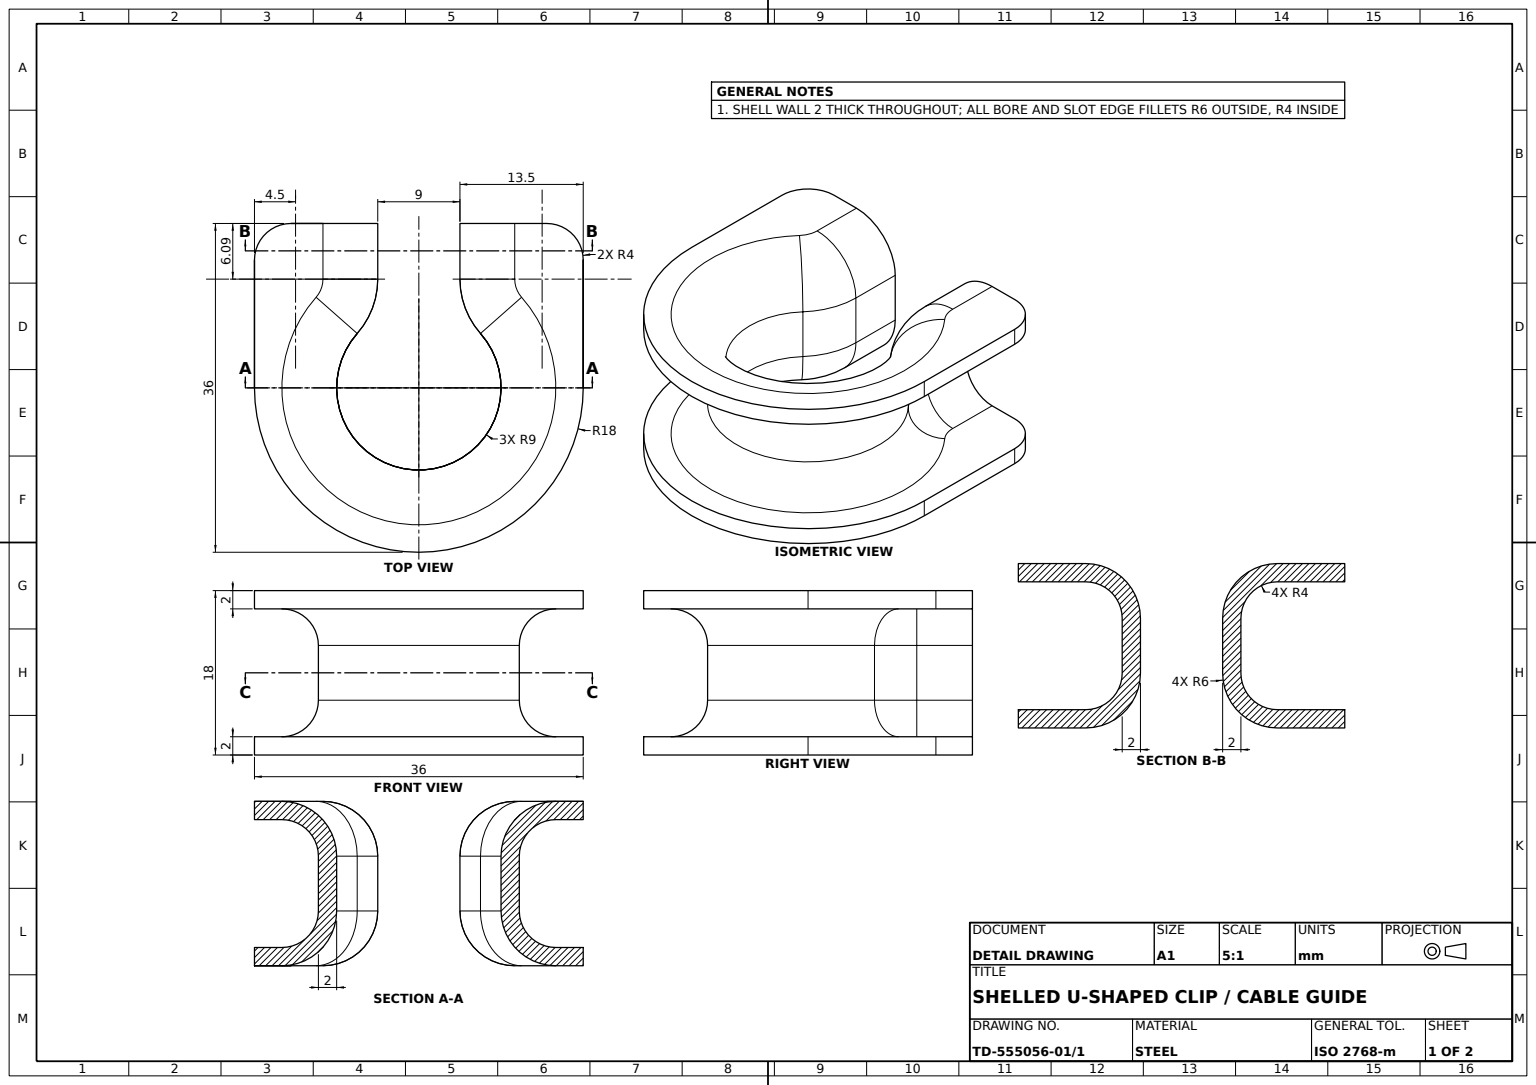
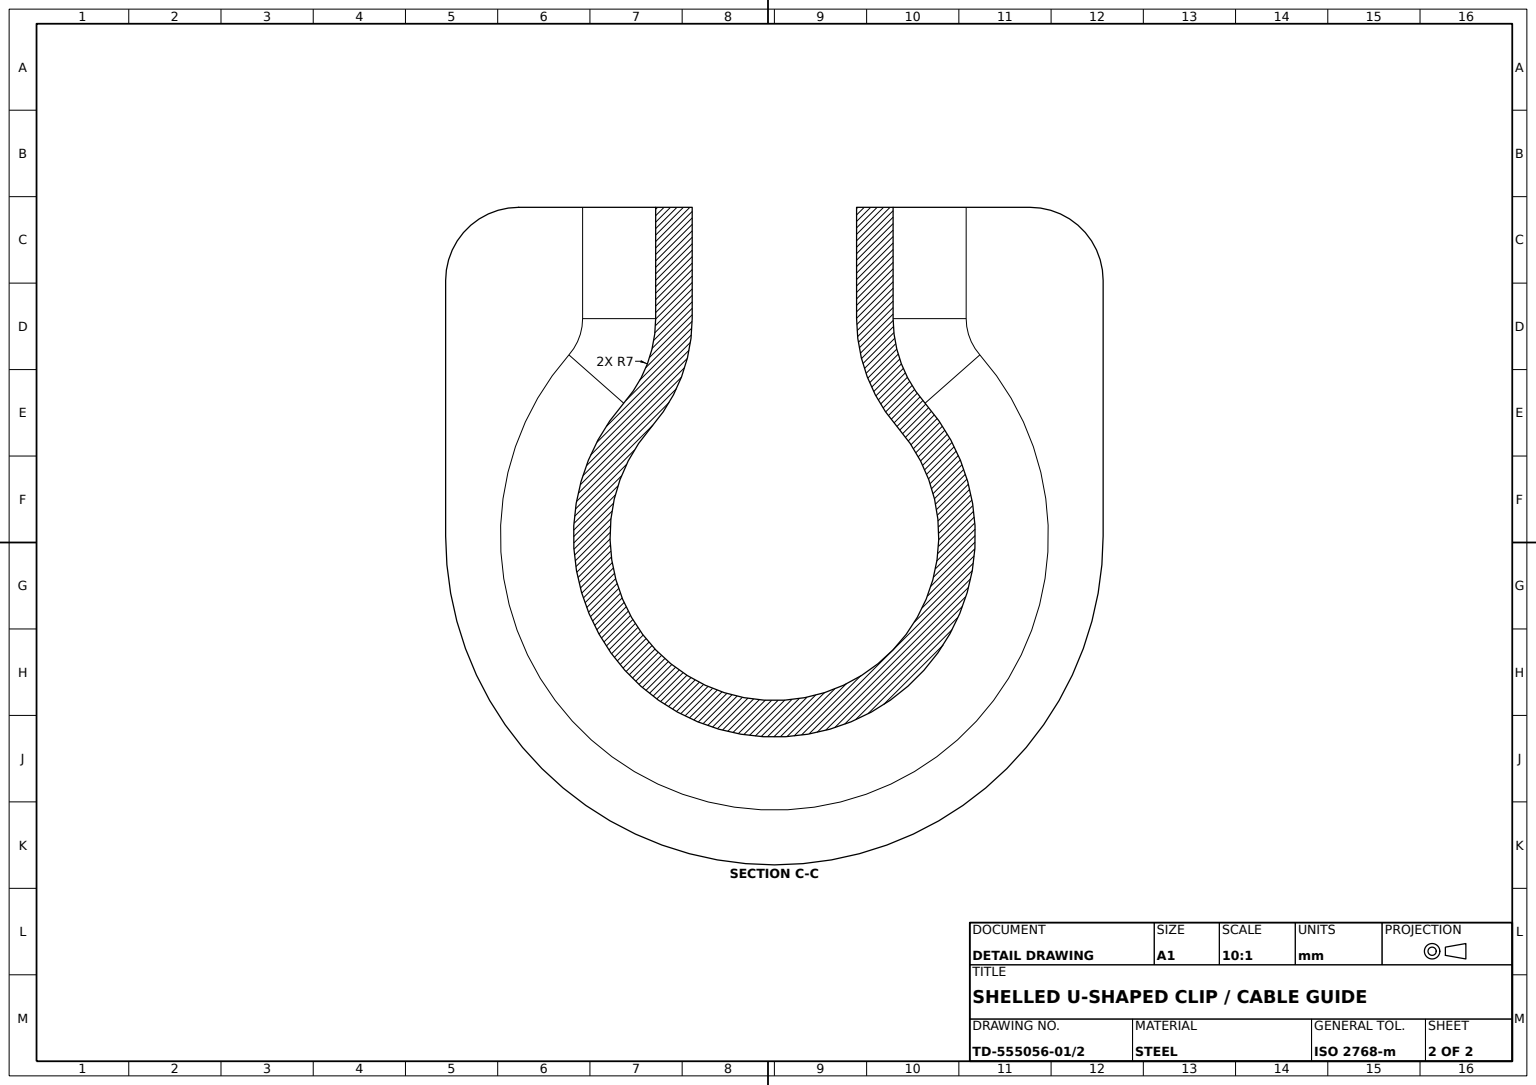
ISO-10303-21;
HEADER;
FILE_DESCRIPTION((''),'2;1');
FILE_NAME('','',(''),(''),'','','');
FILE_SCHEMA(('AUTOMOTIVE_DESIGN'));
ENDSEC;
DATA;
#1=APPLICATION_CONTEXT('');
#2=PRODUCT_CONTEXT('',#1,'mechanical');
#3=PRODUCT('','','',(#2));
#4=PRODUCT_DEFINITION_FORMATION('','',#3);
#5=PRODUCT_DEFINITION_CONTEXT('',#1,'design');
#6=PRODUCT_DEFINITION('','',#4,#5);
#7=PRODUCT_DEFINITION_SHAPE('','',#6);
#8=(LENGTH_UNIT()NAMED_UNIT(*)SI_UNIT(.MILLI.,.METRE.));
#9=(NAMED_UNIT(*)PLANE_ANGLE_UNIT()SI_UNIT($,.RADIAN.));
#10=(NAMED_UNIT(*)SI_UNIT($,.STERADIAN.)SOLID_ANGLE_UNIT());
#11=UNCERTAINTY_MEASURE_WITH_UNIT(LENGTH_MEASURE(1.E-05),#8,'distance_accuracy_value','');
#12=(GEOMETRIC_REPRESENTATION_CONTEXT(3)GLOBAL_UNCERTAINTY_ASSIGNED_CONTEXT((#11))GLOBAL_UNIT_ASSIGNED_CONTEXT((#8,#9,#10))REPRESENTATION_CONTEXT('',''));
#13=CARTESIAN_POINT('',(8.25,-3.,-7.275816));
#14=VERTEX_POINT('',#13);
#15=CARTESIAN_POINT('',(-8.25,-3.,-7.275816));
#16=VERTEX_POINT('',#15);
#17=CARTESIAN_POINT('',(0.,-3.,0.));
#18=DIRECTION('',(0.,-1.,0.));
#19=DIRECTION('',(0.,0.,-1.));
#20=AXIS2_PLACEMENT_3D('',#17,#18,#19);
#21=CIRCLE('',#20,11.);
#22=EDGE_CURVE('',#14,#16,#21,.T.);
#23=ORIENTED_EDGE('',*,*,#22,.F.);
#24=CARTESIAN_POINT('',(8.25,3.,-7.275816));
#25=VERTEX_POINT('',#24);
#26=CARTESIAN_POINT('',(8.25,9.,-7.275816));
#27=VECTOR('',#18,1000.);
#28=LINE('',#26,#27);
#29=EDGE_CURVE('',#25,#14,#28,.T.);
#30=ORIENTED_EDGE('',*,*,#29,.F.);
#31=CARTESIAN_POINT('',(-8.25,3.,-7.275816));
#32=VERTEX_POINT('',#31);
#33=CARTESIAN_POINT('',(0.,3.,0.));
#34=DIRECTION('',(0.,1.,0.));
#35=AXIS2_PLACEMENT_3D('',#33,#34,#19);
#36=CIRCLE('',#35,11.);
#37=EDGE_CURVE('',#32,#25,#36,.T.);
#38=ORIENTED_EDGE('',*,*,#37,.F.);
#39=CARTESIAN_POINT('',(-8.25,9.,-7.275816));
#40=LINE('',#39,#27);
#41=EDGE_CURVE('',#32,#16,#40,.T.);
#42=ORIENTED_EDGE('',*,*,#41,.T.);
#43=EDGE_LOOP('',(#23,#30,#38,#42));
#44=FACE_OUTER_BOUND('',#43,.T.);
#45=CARTESIAN_POINT('',(0.,9.,0.));
#46=AXIS2_PLACEMENT_3D('',#45,#18,#19);
#47=CYLINDRICAL_SURFACE('',#46,11.);
#48=ADVANCED_FACE('',(#44),#47,.T.);
#49=CARTESIAN_POINT('',(4.5,-3.,-11.905881));
#50=VERTEX_POINT('',#49);
#51=CARTESIAN_POINT('',(6.75,-3.,-5.95294));
#52=VERTEX_POINT('',#51);
#53=CARTESIAN_POINT('',(13.5,-3.,-11.905881));
#54=AXIS2_PLACEMENT_3D('',#53,#34,#19);
#55=CIRCLE('',#54,9.);
#56=EDGE_CURVE('',#50,#52,#55,.T.);
#57=ORIENTED_EDGE('',*,*,#56,.T.);
#58=CARTESIAN_POINT('',(6.75,3.,-5.95294));
#59=VERTEX_POINT('',#58);
#60=CARTESIAN_POINT('',(6.75,9.,-5.95294));
#61=LINE('',#60,#27);
#62=EDGE_CURVE('',#59,#52,#61,.T.);
#63=ORIENTED_EDGE('',*,*,#62,.F.);
#64=CARTESIAN_POINT('',(4.5,3.,-11.905881));
#65=VERTEX_POINT('',#64);
#66=CARTESIAN_POINT('',(13.5,3.,-11.905881));
#67=AXIS2_PLACEMENT_3D('',#66,#18,#19);
#68=CIRCLE('',#67,9.);
#69=EDGE_CURVE('',#59,#65,#68,.T.);
#70=ORIENTED_EDGE('',*,*,#69,.T.);
#71=CARTESIAN_POINT('',(4.5,9.,-11.905881));
#72=LINE('',#71,#27);
#73=EDGE_CURVE('',#65,#50,#72,.T.);
#74=ORIENTED_EDGE('',*,*,#73,.T.);
#75=EDGE_LOOP('',(#57,#63,#70,#74));
#76=FACE_OUTER_BOUND('',#75,.T.);
#77=CARTESIAN_POINT('',(13.5,9.,-11.905881));
#78=AXIS2_PLACEMENT_3D('',#77,#18,#19);
#79=CYLINDRICAL_SURFACE('',#78,9.);
#80=ADVANCED_FACE('',(#76),#79,.T.);
#81=CARTESIAN_POINT('',(4.5,-3.,-18.));
#82=VERTEX_POINT('',#81);
#83=DIRECTION('',(0.,0.,1.));
#84=VECTOR('',#83,1000.);
#85=LINE('',#49,#84);
#86=EDGE_CURVE('',#82,#50,#85,.T.);
#87=ORIENTED_EDGE('',*,*,#86,.T.);
#88=ORIENTED_EDGE('',*,*,#73,.F.);
#89=CARTESIAN_POINT('',(4.5,3.,-18.));
#90=VERTEX_POINT('',#89);
#91=VECTOR('',#19,1000.);
#92=LINE('',#89,#91);
#93=EDGE_CURVE('',#65,#90,#92,.T.);
#94=ORIENTED_EDGE('',*,*,#93,.T.);
#95=CARTESIAN_POINT('',(4.5,9.,-18.));
#96=LINE('',#95,#27);
#97=EDGE_CURVE('',#90,#82,#96,.T.);
#98=ORIENTED_EDGE('',*,*,#97,.T.);
#99=EDGE_LOOP('',(#87,#88,#94,#98));
#100=FACE_OUTER_BOUND('',#99,.T.);
#101=DIRECTION('',(1.,0.,0.));
#102=AXIS2_PLACEMENT_3D('',#95,#101,#19);
#103=PLANE('',#102);
#104=ADVANCED_FACE('',(#100),#103,.F.);
#105=CARTESIAN_POINT('',(-4.5,3.,-11.905881));
#106=VERTEX_POINT('',#105);
#107=CARTESIAN_POINT('',(-6.75,3.,-5.95294));
#108=VERTEX_POINT('',#107);
#109=CARTESIAN_POINT('',(-13.5,3.,-11.905881));
#110=AXIS2_PLACEMENT_3D('',#109,#18,#19);
#111=CIRCLE('',#110,9.);
#112=EDGE_CURVE('',#106,#108,#111,.T.);
#113=ORIENTED_EDGE('',*,*,#112,.F.);
#114=CARTESIAN_POINT('',(-10.5,9.,-11.905881));
#115=VERTEX_POINT('',#114);
#116=CARTESIAN_POINT('',(-10.5,3.,-11.905881));
#117=AXIS2_PLACEMENT_3D('',#116,#83,#101);
#118=CIRCLE('',#117,6.);
#119=EDGE_CURVE('',#106,#115,#118,.T.);
#120=ORIENTED_EDGE('',*,*,#119,.T.);
#121=CARTESIAN_POINT('',(-11.25,9.,-9.921567));
#122=VERTEX_POINT('',#121);
#123=CARTESIAN_POINT('',(-13.5,9.,-11.905881));
#124=AXIS2_PLACEMENT_3D('',#123,#34,#19);
#125=CIRCLE('',#124,3.);
#126=EDGE_CURVE('',#122,#115,#125,.T.);
#127=ORIENTED_EDGE('',*,*,#126,.F.);
#128=CARTESIAN_POINT('',(-11.25,3.,-9.921567));
#129=DIRECTION('',(-0.661437828,0.,0.75));
#130=DIRECTION('',(0.75,0.,0.661437828));
#131=AXIS2_PLACEMENT_3D('',#128,#129,#130);
#132=CIRCLE('',#131,6.);
#133=EDGE_CURVE('',#108,#122,#132,.T.);
#134=ORIENTED_EDGE('',*,*,#133,.F.);
#135=EDGE_LOOP('',(#113,#120,#127,#134));
#136=FACE_OUTER_BOUND('',#135,.T.);
#137=TOROIDAL_SURFACE('',#110,3.,6.);
#138=ADVANCED_FACE('',(#136),#137,.T.);
#139=CARTESIAN_POINT('',(10.5,-9.,-11.905881));
#140=VERTEX_POINT('',#139);
#141=CARTESIAN_POINT('',(10.5,-9.,-18.));
#142=VERTEX_POINT('',#141);
#143=LINE('',#141,#91);
#144=EDGE_CURVE('',#140,#142,#143,.T.);
#145=ORIENTED_EDGE('',*,*,#144,.F.);
#146=CARTESIAN_POINT('',(10.5,-3.,-11.905881));
#147=DIRECTION('',(-1.,0.,0.));
#148=AXIS2_PLACEMENT_3D('',#146,#19,#147);
#149=CIRCLE('',#148,6.);
#150=EDGE_CURVE('',#140,#50,#149,.T.);
#151=ORIENTED_EDGE('',*,*,#150,.T.);
#152=ORIENTED_EDGE('',*,*,#86,.F.);
#153=CARTESIAN_POINT('',(10.5,-3.,-18.));
#154=AXIS2_PLACEMENT_3D('',#153,#19,#101);
#155=CIRCLE('',#154,6.);
#156=EDGE_CURVE('',#142,#82,#155,.T.);
#157=ORIENTED_EDGE('',*,*,#156,.F.);
#158=EDGE_LOOP('',(#145,#151,#152,#157));
#159=FACE_OUTER_BOUND('',#158,.T.);
#160=AXIS2_PLACEMENT_3D('',#153,#19,#147);
#161=CYLINDRICAL_SURFACE('',#160,6.);
#162=ADVANCED_FACE('',(#159),#161,.T.);
#163=CARTESIAN_POINT('',(-18.,7.,0.));
#164=VERTEX_POINT('',#163);
#165=CARTESIAN_POINT('',(18.,7.,0.));
#166=VERTEX_POINT('',#165);
#167=CARTESIAN_POINT('',(0.,7.,0.));
#168=AXIS2_PLACEMENT_3D('',#167,#34,#19);
#169=CIRCLE('',#168,18.);
#170=EDGE_CURVE('',#164,#166,#169,.T.);
#171=ORIENTED_EDGE('',*,*,#170,.T.);
#172=CARTESIAN_POINT('',(18.,9.,0.));
#173=VERTEX_POINT('',#172);
#174=LINE('',#172,#27);
#175=EDGE_CURVE('',#173,#166,#174,.T.);
#176=ORIENTED_EDGE('',*,*,#175,.F.);
#177=CARTESIAN_POINT('',(-18.,9.,0.));
#178=VERTEX_POINT('',#177);
#179=AXIS2_PLACEMENT_3D('',#45,#34,#83);
#180=CIRCLE('',#179,18.);
#181=EDGE_CURVE('',#178,#173,#180,.T.);
#182=ORIENTED_EDGE('',*,*,#181,.F.);
#183=LINE('',#177,#27);
#184=EDGE_CURVE('',#178,#164,#183,.T.);
#185=ORIENTED_EDGE('',*,*,#184,.T.);
#186=EDGE_LOOP('',(#171,#176,#182,#185));
#187=FACE_OUTER_BOUND('',#186,.T.);
#188=CYLINDRICAL_SURFACE('',#46,18.);
#189=ADVANCED_FACE('',(#187),#188,.T.);
#190=CARTESIAN_POINT('',(11.25,7.,-9.921567));
#191=VERTEX_POINT('',#190);
#192=CARTESIAN_POINT('',(-11.25,7.,-9.921567));
#193=VERTEX_POINT('',#192);
#194=AXIS2_PLACEMENT_3D('',#167,#18,#19);
#195=CIRCLE('',#194,15.);
#196=EDGE_CURVE('',#191,#193,#195,.T.);
#197=ORIENTED_EDGE('',*,*,#196,.T.);
#198=CIRCLE('',#131,4.);
#199=EDGE_CURVE('',#32,#193,#198,.T.);
#200=ORIENTED_EDGE('',*,*,#199,.F.);
#201=ORIENTED_EDGE('',*,*,#37,.T.);
#202=CARTESIAN_POINT('',(11.25,3.,-9.921567));
#203=DIRECTION('',(-0.661437828,0.,-0.75));
#204=DIRECTION('',(0.75,0.,-0.661437828));
#205=AXIS2_PLACEMENT_3D('',#202,#203,#204);
#206=CIRCLE('',#205,4.);
#207=EDGE_CURVE('',#25,#191,#206,.T.);
#208=ORIENTED_EDGE('',*,*,#207,.T.);
#209=EDGE_LOOP('',(#197,#200,#201,#208));
#210=FACE_OUTER_BOUND('',#209,.T.);
#211=AXIS2_PLACEMENT_3D('',#33,#18,#19);
#212=TOROIDAL_SURFACE('',#211,15.,4.);
#213=ADVANCED_FACE('',(#210),#212,.F.);
#214=CARTESIAN_POINT('',(6.5,3.,-11.905881));
#215=VERTEX_POINT('',#214);
#216=CARTESIAN_POINT('',(10.5,7.,-11.905881));
#217=VERTEX_POINT('',#216);
#218=CARTESIAN_POINT('',(10.5,3.,-11.905881));
#219=AXIS2_PLACEMENT_3D('',#218,#19,#101);
#220=CIRCLE('',#219,4.);
#221=EDGE_CURVE('',#215,#217,#220,.T.);
#222=ORIENTED_EDGE('',*,*,#221,.T.);
#223=CARTESIAN_POINT('',(13.5,7.,-11.905881));
#224=AXIS2_PLACEMENT_3D('',#223,#34,#19);
#225=CIRCLE('',#224,3.);
#226=EDGE_CURVE('',#217,#191,#225,.T.);
#227=ORIENTED_EDGE('',*,*,#226,.T.);
#228=ORIENTED_EDGE('',*,*,#207,.F.);
#229=CIRCLE('',#67,7.);
#230=EDGE_CURVE('',#25,#215,#229,.T.);
#231=ORIENTED_EDGE('',*,*,#230,.T.);
#232=EDGE_LOOP('',(#222,#227,#228,#231));
#233=FACE_OUTER_BOUND('',#232,.T.);
#234=TOROIDAL_SURFACE('',#67,3.,4.);
#235=ADVANCED_FACE('',(#233),#234,.F.);
#236=CARTESIAN_POINT('',(-6.5,-3.,-18.));
#237=VERTEX_POINT('',#236);
#238=CARTESIAN_POINT('',(-10.5,-7.,-18.));
#239=VERTEX_POINT('',#238);
#240=CARTESIAN_POINT('',(-10.5,-3.,-18.));
#241=AXIS2_PLACEMENT_3D('',#240,#19,#101);
#242=CIRCLE('',#241,4.);
#243=EDGE_CURVE('',#237,#239,#242,.T.);
#244=ORIENTED_EDGE('',*,*,#243,.F.);
#245=CARTESIAN_POINT('',(-6.5,3.,-18.));
#246=VERTEX_POINT('',#245);
#247=CARTESIAN_POINT('',(-6.5,9.,-18.));
#248=LINE('',#247,#27);
#249=EDGE_CURVE('',#246,#237,#248,.T.);
#250=ORIENTED_EDGE('',*,*,#249,.F.);
#251=CARTESIAN_POINT('',(-10.5,7.,-18.));
#252=VERTEX_POINT('',#251);
#253=CARTESIAN_POINT('',(-10.5,3.,-18.));
#254=AXIS2_PLACEMENT_3D('',#253,#19,#101);
#255=CIRCLE('',#254,4.);
#256=EDGE_CURVE('',#252,#246,#255,.T.);
#257=ORIENTED_EDGE('',*,*,#256,.F.);
#258=CARTESIAN_POINT('',(-14.,7.,-18.));
#259=VERTEX_POINT('',#258);
#260=CARTESIAN_POINT('',(-13.5,7.,-18.));
#261=VECTOR('',#147,1000.);
#262=LINE('',#260,#261);
#263=EDGE_CURVE('',#252,#259,#262,.T.);
#264=ORIENTED_EDGE('',*,*,#263,.T.);
#265=CARTESIAN_POINT('',(-14.,9.,-18.));
#266=VERTEX_POINT('',#265);
#267=LINE('',#265,#27);
#268=EDGE_CURVE('',#266,#259,#267,.T.);
#269=ORIENTED_EDGE('',*,*,#268,.F.);
#270=CARTESIAN_POINT('',(-10.5,9.,-18.));
#271=VERTEX_POINT('',#270);
#272=LINE('',#265,#261);
#273=EDGE_CURVE('',#271,#266,#272,.T.);
#274=ORIENTED_EDGE('',*,*,#273,.F.);
#275=CARTESIAN_POINT('',(-4.5,3.,-18.));
#276=VERTEX_POINT('',#275);
#277=CIRCLE('',#254,6.);
#278=EDGE_CURVE('',#271,#276,#277,.T.);
#279=ORIENTED_EDGE('',*,*,#278,.T.);
#280=CARTESIAN_POINT('',(-4.5,-3.,-18.));
#281=VERTEX_POINT('',#280);
#282=CARTESIAN_POINT('',(-4.5,9.,-18.));
#283=LINE('',#282,#27);
#284=EDGE_CURVE('',#276,#281,#283,.T.);
#285=ORIENTED_EDGE('',*,*,#284,.T.);
#286=CARTESIAN_POINT('',(-10.5,-9.,-18.));
#287=VERTEX_POINT('',#286);
#288=CIRCLE('',#241,6.);
#289=EDGE_CURVE('',#281,#287,#288,.T.);
#290=ORIENTED_EDGE('',*,*,#289,.T.);
#291=CARTESIAN_POINT('',(-14.,-9.,-18.));
#292=VERTEX_POINT('',#291);
#293=LINE('',#291,#261);
#294=EDGE_CURVE('',#287,#292,#293,.T.);
#295=ORIENTED_EDGE('',*,*,#294,.T.);
#296=CARTESIAN_POINT('',(-14.,-7.,-18.));
#297=VERTEX_POINT('',#296);
#298=EDGE_CURVE('',#297,#292,#267,.T.);
#299=ORIENTED_EDGE('',*,*,#298,.F.);
#300=CARTESIAN_POINT('',(-13.5,-7.,-18.));
#301=LINE('',#300,#261);
#302=EDGE_CURVE('',#239,#297,#301,.T.);
#303=ORIENTED_EDGE('',*,*,#302,.F.);
#304=EDGE_LOOP('',(#244,#250,#257,#264,#269,#274,#279,#285,#290,#295,#299,#303));
#305=FACE_OUTER_BOUND('',#304,.T.);
#306=AXIS2_PLACEMENT_3D('',#265,#83,#101);
#307=PLANE('',#306);
#308=ADVANCED_FACE('',(#305),#307,.F.);
#309=CARTESIAN_POINT('',(-6.5,3.,-11.905881));
#310=VERTEX_POINT('',#309);
#311=CIRCLE('',#110,7.);
#312=EDGE_CURVE('',#310,#32,#311,.T.);
#313=ORIENTED_EDGE('',*,*,#312,.F.);
#314=CARTESIAN_POINT('',(-6.5,-3.,-11.905881));
#315=VERTEX_POINT('',#314);
#316=CARTESIAN_POINT('',(-6.5,9.,-11.905881));
#317=LINE('',#316,#27);
#318=EDGE_CURVE('',#310,#315,#317,.T.);
#319=ORIENTED_EDGE('',*,*,#318,.T.);
#320=CARTESIAN_POINT('',(-13.5,-3.,-11.905881));
#321=AXIS2_PLACEMENT_3D('',#320,#34,#19);
#322=CIRCLE('',#321,7.);
#323=EDGE_CURVE('',#16,#315,#322,.T.);
#324=ORIENTED_EDGE('',*,*,#323,.F.);
#325=ORIENTED_EDGE('',*,*,#41,.F.);
#326=EDGE_LOOP('',(#313,#319,#324,#325));
#327=FACE_OUTER_BOUND('',#326,.T.);
#328=AXIS2_PLACEMENT_3D('',#123,#18,#19);
#329=CYLINDRICAL_SURFACE('',#328,7.);
#330=ADVANCED_FACE('',(#327),#329,.F.);
#331=CARTESIAN_POINT('',(10.5,-7.,-11.905881));
#332=VERTEX_POINT('',#331);
#333=CARTESIAN_POINT('',(10.5,-7.,-18.));
#334=VERTEX_POINT('',#333);
#335=LINE('',#331,#91);
#336=EDGE_CURVE('',#332,#334,#335,.T.);
#337=ORIENTED_EDGE('',*,*,#336,.F.);
#338=CARTESIAN_POINT('',(11.25,-7.,-9.921567));
#339=VERTEX_POINT('',#338);
#340=CARTESIAN_POINT('',(13.5,-7.,-11.905881));
#341=AXIS2_PLACEMENT_3D('',#340,#18,#19);
#342=CIRCLE('',#341,3.);
#343=EDGE_CURVE('',#339,#332,#342,.T.);
#344=ORIENTED_EDGE('',*,*,#343,.F.);
#345=CARTESIAN_POINT('',(-11.25,-7.,-9.921567));
#346=VERTEX_POINT('',#345);
#347=CARTESIAN_POINT('',(0.,-7.,0.));
#348=AXIS2_PLACEMENT_3D('',#347,#34,#19);
#349=CIRCLE('',#348,15.);
#350=EDGE_CURVE('',#346,#339,#349,.T.);
#351=ORIENTED_EDGE('',*,*,#350,.F.);
#352=CARTESIAN_POINT('',(-10.5,-7.,-11.905881));
#353=VERTEX_POINT('',#352);
#354=CARTESIAN_POINT('',(-13.5,-7.,-11.905881));
#355=AXIS2_PLACEMENT_3D('',#354,#18,#19);
#356=CIRCLE('',#355,3.);
#357=EDGE_CURVE('',#353,#346,#356,.T.);
#358=ORIENTED_EDGE('',*,*,#357,.F.);
#359=LINE('',#352,#84);
#360=EDGE_CURVE('',#239,#353,#359,.T.);
#361=ORIENTED_EDGE('',*,*,#360,.F.);
#362=ORIENTED_EDGE('',*,*,#302,.T.);
#363=CARTESIAN_POINT('',(-18.,-7.,-14.));
#364=VERTEX_POINT('',#363);
#365=CARTESIAN_POINT('',(-14.,-7.,-14.));
#366=AXIS2_PLACEMENT_3D('',#365,#34,#19);
#367=CIRCLE('',#366,4.);
#368=EDGE_CURVE('',#297,#364,#367,.T.);
#369=ORIENTED_EDGE('',*,*,#368,.T.);
#370=CARTESIAN_POINT('',(-18.,-7.,0.));
#371=VERTEX_POINT('',#370);
#372=CARTESIAN_POINT('',(-18.,-7.,-11.905881));
#373=LINE('',#372,#84);
#374=EDGE_CURVE('',#364,#371,#373,.T.);
#375=ORIENTED_EDGE('',*,*,#374,.T.);
#376=CARTESIAN_POINT('',(18.,-7.,0.));
#377=VERTEX_POINT('',#376);
#378=CIRCLE('',#348,18.);
#379=EDGE_CURVE('',#371,#377,#378,.T.);
#380=ORIENTED_EDGE('',*,*,#379,.T.);
#381=CARTESIAN_POINT('',(18.,-7.,-14.));
#382=VERTEX_POINT('',#381);
#383=CARTESIAN_POINT('',(18.,-7.,-11.905881));
#384=LINE('',#383,#91);
#385=EDGE_CURVE('',#377,#382,#384,.T.);
#386=ORIENTED_EDGE('',*,*,#385,.T.);
#387=CARTESIAN_POINT('',(14.,-7.,-18.));
#388=VERTEX_POINT('',#387);
#389=CARTESIAN_POINT('',(14.,-7.,-14.));
#390=AXIS2_PLACEMENT_3D('',#389,#34,#19);
#391=CIRCLE('',#390,4.);
#392=EDGE_CURVE('',#382,#388,#391,.T.);
#393=ORIENTED_EDGE('',*,*,#392,.T.);
#394=EDGE_CURVE('',#388,#334,#301,.T.);
#395=ORIENTED_EDGE('',*,*,#394,.T.);
#396=EDGE_LOOP('',(#337,#344,#351,#358,#361,#362,#369,#375,#380,#386,#393,#395));
#397=FACE_OUTER_BOUND('',#396,.T.);
#398=PLANE('',#355);
#399=ADVANCED_FACE('',(#397),#398,.F.);
#400=CARTESIAN_POINT('',(-10.5,-9.,-11.905881));
#401=VERTEX_POINT('',#400);
#402=LINE('',#400,#84);
#403=EDGE_CURVE('',#287,#401,#402,.T.);
#404=ORIENTED_EDGE('',*,*,#403,.F.);
#405=ORIENTED_EDGE('',*,*,#289,.F.);
#406=CARTESIAN_POINT('',(-4.5,-3.,-11.905881));
#407=VERTEX_POINT('',#406);
#408=LINE('',#280,#91);
#409=EDGE_CURVE('',#407,#281,#408,.T.);
#410=ORIENTED_EDGE('',*,*,#409,.F.);
#411=CARTESIAN_POINT('',(-10.5,-3.,-11.905881));
#412=AXIS2_PLACEMENT_3D('',#411,#83,#101);
#413=CIRCLE('',#412,6.);
#414=EDGE_CURVE('',#401,#407,#413,.T.);
#415=ORIENTED_EDGE('',*,*,#414,.F.);
#416=EDGE_LOOP('',(#404,#405,#410,#415));
#417=FACE_OUTER_BOUND('',#416,.T.);
#418=AXIS2_PLACEMENT_3D('',#240,#83,#101);
#419=CYLINDRICAL_SURFACE('',#418,6.);
#420=ADVANCED_FACE('',(#417),#419,.T.);
#421=ORIENTED_EDGE('',*,*,#69,.F.);
#422=CARTESIAN_POINT('',(11.25,9.,-9.921567));
#423=VERTEX_POINT('',#422);
#424=DIRECTION('',(-0.75,0.,0.661437828));
#425=AXIS2_PLACEMENT_3D('',#202,#203,#424);
#426=CIRCLE('',#425,6.);
#427=EDGE_CURVE('',#59,#423,#426,.T.);
#428=ORIENTED_EDGE('',*,*,#427,.T.);
#429=CARTESIAN_POINT('',(10.5,9.,-11.905881));
#430=VERTEX_POINT('',#429);
#431=AXIS2_PLACEMENT_3D('',#77,#34,#19);
#432=CIRCLE('',#431,3.);
#433=EDGE_CURVE('',#430,#423,#432,.T.);
#434=ORIENTED_EDGE('',*,*,#433,.F.);
#435=AXIS2_PLACEMENT_3D('',#218,#19,#147);
#436=CIRCLE('',#435,6.);
#437=EDGE_CURVE('',#65,#430,#436,.T.);
#438=ORIENTED_EDGE('',*,*,#437,.F.);
#439=EDGE_LOOP('',(#421,#428,#434,#438));
#440=FACE_OUTER_BOUND('',#439,.T.);
#441=TOROIDAL_SURFACE('',#67,3.,6.);
#442=ADVANCED_FACE('',(#440),#441,.T.);
#443=CARTESIAN_POINT('',(10.5,9.,-18.));
#444=VERTEX_POINT('',#443);
#445=LINE('',#429,#84);
#446=EDGE_CURVE('',#444,#430,#445,.T.);
#447=ORIENTED_EDGE('',*,*,#446,.F.);
#448=CARTESIAN_POINT('',(10.5,3.,-18.));
#449=AXIS2_PLACEMENT_3D('',#448,#19,#101);
#450=CIRCLE('',#449,6.);
#451=EDGE_CURVE('',#90,#444,#450,.T.);
#452=ORIENTED_EDGE('',*,*,#451,.F.);
#453=ORIENTED_EDGE('',*,*,#93,.F.);
#454=ORIENTED_EDGE('',*,*,#437,.T.);
#455=EDGE_LOOP('',(#447,#452,#453,#454));
#456=FACE_OUTER_BOUND('',#455,.T.);
#457=AXIS2_PLACEMENT_3D('',#218,#83,#101);
#458=CYLINDRICAL_SURFACE('',#457,6.);
#459=ADVANCED_FACE('',(#456),#458,.T.);
#460=ORIENTED_EDGE('',*,*,#385,.F.);
#461=CARTESIAN_POINT('',(18.,-9.,0.));
#462=VERTEX_POINT('',#461);
#463=EDGE_CURVE('',#377,#462,#174,.T.);
#464=ORIENTED_EDGE('',*,*,#463,.T.);
#465=CARTESIAN_POINT('',(18.,-9.,-14.));
#466=VERTEX_POINT('',#465);
#467=LINE('',#465,#91);
#468=EDGE_CURVE('',#462,#466,#467,.T.);
#469=ORIENTED_EDGE('',*,*,#468,.T.);
#470=CARTESIAN_POINT('',(18.,9.,-14.));
#471=LINE('',#470,#27);
#472=EDGE_CURVE('',#382,#466,#471,.T.);
#473=ORIENTED_EDGE('',*,*,#472,.F.);
#474=EDGE_LOOP('',(#460,#464,#469,#473));
#475=FACE_OUTER_BOUND('',#474,.T.);
#476=AXIS2_PLACEMENT_3D('',#470,#147,#83);
#477=PLANE('',#476);
#478=ADVANCED_FACE('',(#475),#477,.F.);
#479=CARTESIAN_POINT('',(10.5,7.,-18.));
#480=VERTEX_POINT('',#479);
#481=LINE('',#216,#84);
#482=EDGE_CURVE('',#480,#217,#481,.T.);
#483=ORIENTED_EDGE('',*,*,#482,.T.);
#484=ORIENTED_EDGE('',*,*,#221,.F.);
#485=CARTESIAN_POINT('',(6.5,3.,-18.));
#486=VERTEX_POINT('',#485);
#487=LINE('',#485,#91);
#488=EDGE_CURVE('',#215,#486,#487,.T.);
#489=ORIENTED_EDGE('',*,*,#488,.T.);
#490=CIRCLE('',#449,4.);
#491=EDGE_CURVE('',#486,#480,#490,.T.);
#492=ORIENTED_EDGE('',*,*,#491,.T.);
#493=EDGE_LOOP('',(#483,#484,#489,#492));
#494=FACE_OUTER_BOUND('',#493,.T.);
#495=CYLINDRICAL_SURFACE('',#457,4.);
#496=ADVANCED_FACE('',(#494),#495,.F.);
#497=CARTESIAN_POINT('',(-6.75,-3.,-5.95294));
#498=VERTEX_POINT('',#497);
#499=CIRCLE('',#20,9.);
#500=EDGE_CURVE('',#52,#498,#499,.T.);
#501=ORIENTED_EDGE('',*,*,#500,.F.);
#502=CARTESIAN_POINT('',(11.25,-9.,-9.921567));
#503=VERTEX_POINT('',#502);
#504=CARTESIAN_POINT('',(11.25,-3.,-9.921567));
#505=AXIS2_PLACEMENT_3D('',#504,#203,#424);
#506=CIRCLE('',#505,6.);
#507=EDGE_CURVE('',#503,#52,#506,.T.);
#508=ORIENTED_EDGE('',*,*,#507,.F.);
#509=CARTESIAN_POINT('',(-11.25,-9.,-9.921567));
#510=VERTEX_POINT('',#509);
#511=CARTESIAN_POINT('',(0.,-9.,0.));
#512=AXIS2_PLACEMENT_3D('',#511,#34,#19);
#513=CIRCLE('',#512,15.);
#514=EDGE_CURVE('',#510,#503,#513,.T.);
#515=ORIENTED_EDGE('',*,*,#514,.F.);
#516=CARTESIAN_POINT('',(-11.25,-3.,-9.921567));
#517=AXIS2_PLACEMENT_3D('',#516,#129,#130);
#518=CIRCLE('',#517,6.);
#519=EDGE_CURVE('',#510,#498,#518,.T.);
#520=ORIENTED_EDGE('',*,*,#519,.T.);
#521=EDGE_LOOP('',(#501,#508,#515,#520));
#522=FACE_OUTER_BOUND('',#521,.T.);
#523=TOROIDAL_SURFACE('',#20,15.,6.);
#524=ADVANCED_FACE('',(#522),#523,.T.);
#525=CARTESIAN_POINT('',(-18.,9.,-14.));
#526=VERTEX_POINT('',#525);
#527=CARTESIAN_POINT('',(-18.,7.,-14.));
#528=VERTEX_POINT('',#527);
#529=LINE('',#525,#27);
#530=EDGE_CURVE('',#526,#528,#529,.T.);
#531=ORIENTED_EDGE('',*,*,#530,.F.);
#532=CARTESIAN_POINT('',(-14.,9.,-14.));
#533=AXIS2_PLACEMENT_3D('',#532,#34,#83);
#534=CIRCLE('',#533,4.);
#535=EDGE_CURVE('',#266,#526,#534,.T.);
#536=ORIENTED_EDGE('',*,*,#535,.F.);
#537=ORIENTED_EDGE('',*,*,#268,.T.);
#538=CARTESIAN_POINT('',(-14.,7.,-14.));
#539=AXIS2_PLACEMENT_3D('',#538,#34,#19);
#540=CIRCLE('',#539,4.);
#541=EDGE_CURVE('',#259,#528,#540,.T.);
#542=ORIENTED_EDGE('',*,*,#541,.T.);
#543=EDGE_LOOP('',(#531,#536,#537,#542));
#544=FACE_OUTER_BOUND('',#543,.T.);
#545=AXIS2_PLACEMENT_3D('',#532,#18,#19);
#546=CYLINDRICAL_SURFACE('',#545,4.);
#547=ADVANCED_FACE('',(#544),#546,.T.);
#548=CARTESIAN_POINT('',(6.5,-3.,-11.905881));
#549=VERTEX_POINT('',#548);
#550=CIRCLE('',#54,7.);
#551=EDGE_CURVE('',#549,#14,#550,.T.);
#552=ORIENTED_EDGE('',*,*,#551,.T.);
#553=AXIS2_PLACEMENT_3D('',#504,#203,#204);
#554=CIRCLE('',#553,4.);
#555=EDGE_CURVE('',#339,#14,#554,.T.);
#556=ORIENTED_EDGE('',*,*,#555,.F.);
#557=ORIENTED_EDGE('',*,*,#343,.T.);
#558=CIRCLE('',#148,4.);
#559=EDGE_CURVE('',#332,#549,#558,.T.);
#560=ORIENTED_EDGE('',*,*,#559,.T.);
#561=EDGE_LOOP('',(#552,#556,#557,#560));
#562=FACE_OUTER_BOUND('',#561,.T.);
#563=AXIS2_PLACEMENT_3D('',#53,#18,#19);
#564=TOROIDAL_SURFACE('',#563,3.,4.);
#565=ADVANCED_FACE('',(#562),#564,.F.);
#566=CARTESIAN_POINT('',(14.,-9.,-18.));
#567=VERTEX_POINT('',#566);
#568=CARTESIAN_POINT('',(4.5,-9.,-18.));
#569=LINE('',#568,#261);
#570=EDGE_CURVE('',#567,#142,#569,.T.);
#571=ORIENTED_EDGE('',*,*,#570,.F.);
#572=CARTESIAN_POINT('',(14.,-9.,-14.));
#573=AXIS2_PLACEMENT_3D('',#572,#34,#83);
#574=CIRCLE('',#573,4.);
#575=EDGE_CURVE('',#466,#567,#574,.T.);
#576=ORIENTED_EDGE('',*,*,#575,.F.);
#577=ORIENTED_EDGE('',*,*,#468,.F.);
#578=CARTESIAN_POINT('',(-18.,-9.,0.));
#579=VERTEX_POINT('',#578);
#580=AXIS2_PLACEMENT_3D('',#511,#34,#83);
#581=CIRCLE('',#580,18.);
#582=EDGE_CURVE('',#579,#462,#581,.T.);
#583=ORIENTED_EDGE('',*,*,#582,.F.);
#584=CARTESIAN_POINT('',(-18.,-9.,-14.));
#585=VERTEX_POINT('',#584);
#586=LINE('',#584,#84);
#587=EDGE_CURVE('',#585,#579,#586,.T.);
#588=ORIENTED_EDGE('',*,*,#587,.F.);
#589=CARTESIAN_POINT('',(-14.,-9.,-14.));
#590=AXIS2_PLACEMENT_3D('',#589,#34,#83);
#591=CIRCLE('',#590,4.);
#592=EDGE_CURVE('',#292,#585,#591,.T.);
#593=ORIENTED_EDGE('',*,*,#592,.F.);
#594=ORIENTED_EDGE('',*,*,#294,.F.);
#595=ORIENTED_EDGE('',*,*,#403,.T.);
#596=CARTESIAN_POINT('',(-13.5,-9.,-11.905881));
#597=AXIS2_PLACEMENT_3D('',#596,#18,#19);
#598=CIRCLE('',#597,3.);
#599=EDGE_CURVE('',#401,#510,#598,.T.);
#600=ORIENTED_EDGE('',*,*,#599,.T.);
#601=ORIENTED_EDGE('',*,*,#514,.T.);
#602=CARTESIAN_POINT('',(13.5,-9.,-11.905881));
#603=AXIS2_PLACEMENT_3D('',#602,#18,#19);
#604=CIRCLE('',#603,3.);
#605=EDGE_CURVE('',#503,#140,#604,.T.);
#606=ORIENTED_EDGE('',*,*,#605,.T.);
#607=ORIENTED_EDGE('',*,*,#144,.T.);
#608=EDGE_LOOP('',(#571,#576,#577,#583,#588,#593,#594,#595,#600,#601,#606,#607));
#609=FACE_OUTER_BOUND('',#608,.T.);
#610=PLANE('',#597);
#611=ADVANCED_FACE('',(#609),#610,.T.);
#612=ORIENTED_EDGE('',*,*,#126,.T.);
#613=LINE('',#114,#91);
#614=EDGE_CURVE('',#115,#271,#613,.T.);
#615=ORIENTED_EDGE('',*,*,#614,.T.);
#616=ORIENTED_EDGE('',*,*,#273,.T.);
#617=ORIENTED_EDGE('',*,*,#535,.T.);
#618=LINE('',#525,#84);
#619=EDGE_CURVE('',#526,#178,#618,.T.);
#620=ORIENTED_EDGE('',*,*,#619,.T.);
#621=ORIENTED_EDGE('',*,*,#181,.T.);
#622=VERTEX_POINT('',#470);
#623=LINE('',#470,#91);
#624=EDGE_CURVE('',#173,#622,#623,.T.);
#625=ORIENTED_EDGE('',*,*,#624,.T.);
#626=CARTESIAN_POINT('',(14.,9.,-18.));
#627=VERTEX_POINT('',#626);
#628=CARTESIAN_POINT('',(14.,9.,-14.));
#629=AXIS2_PLACEMENT_3D('',#628,#34,#83);
#630=CIRCLE('',#629,4.);
#631=EDGE_CURVE('',#622,#627,#630,.T.);
#632=ORIENTED_EDGE('',*,*,#631,.T.);
#633=LINE('',#95,#261);
#634=EDGE_CURVE('',#627,#444,#633,.T.);
#635=ORIENTED_EDGE('',*,*,#634,.T.);
#636=ORIENTED_EDGE('',*,*,#446,.T.);
#637=ORIENTED_EDGE('',*,*,#433,.T.);
#638=CIRCLE('',#46,15.);
#639=EDGE_CURVE('',#423,#122,#638,.T.);
#640=ORIENTED_EDGE('',*,*,#639,.T.);
#641=EDGE_LOOP('',(#612,#615,#616,#617,#620,#621,#625,#632,#635,#636,#637,#640));
#642=FACE_OUTER_BOUND('',#641,.T.);
#643=PLANE('',#328);
#644=ADVANCED_FACE('',(#642),#643,.F.);
#645=ORIENTED_EDGE('',*,*,#559,.F.);
#646=ORIENTED_EDGE('',*,*,#336,.T.);
#647=CARTESIAN_POINT('',(6.5,-3.,-18.));
#648=VERTEX_POINT('',#647);
#649=CIRCLE('',#154,4.);
#650=EDGE_CURVE('',#334,#648,#649,.T.);
#651=ORIENTED_EDGE('',*,*,#650,.T.);
#652=LINE('',#647,#84);
#653=EDGE_CURVE('',#648,#549,#652,.T.);
#654=ORIENTED_EDGE('',*,*,#653,.T.);
#655=EDGE_LOOP('',(#645,#646,#651,#654));
#656=FACE_OUTER_BOUND('',#655,.T.);
#657=CYLINDRICAL_SURFACE('',#160,4.);
#658=ADVANCED_FACE('',(#656),#657,.F.);
#659=ORIENTED_EDGE('',*,*,#507,.T.);
#660=ORIENTED_EDGE('',*,*,#56,.F.);
#661=ORIENTED_EDGE('',*,*,#150,.F.);
#662=ORIENTED_EDGE('',*,*,#605,.F.);
#663=EDGE_LOOP('',(#659,#660,#661,#662));
#664=FACE_OUTER_BOUND('',#663,.T.);
#665=TOROIDAL_SURFACE('',#563,3.,6.);
#666=ADVANCED_FACE('',(#664),#665,.T.);
#667=CARTESIAN_POINT('',(18.,7.,-14.));
#668=VERTEX_POINT('',#667);
#669=EDGE_CURVE('',#622,#668,#471,.T.);
#670=ORIENTED_EDGE('',*,*,#669,.F.);
#671=ORIENTED_EDGE('',*,*,#624,.F.);
#672=ORIENTED_EDGE('',*,*,#175,.T.);
#673=CARTESIAN_POINT('',(18.,7.,-11.905881));
#674=LINE('',#673,#91);
#675=EDGE_CURVE('',#166,#668,#674,.T.);
#676=ORIENTED_EDGE('',*,*,#675,.T.);
#677=EDGE_LOOP('',(#670,#671,#672,#676));
#678=FACE_OUTER_BOUND('',#677,.T.);
#679=ADVANCED_FACE('',(#678),#477,.F.);
#680=ORIENTED_EDGE('',*,*,#551,.F.);
#681=CARTESIAN_POINT('',(6.5,9.,-11.905881));
#682=LINE('',#681,#27);
#683=EDGE_CURVE('',#215,#549,#682,.T.);
#684=ORIENTED_EDGE('',*,*,#683,.F.);
#685=ORIENTED_EDGE('',*,*,#230,.F.);
#686=ORIENTED_EDGE('',*,*,#29,.T.);
#687=EDGE_LOOP('',(#680,#684,#685,#686));
#688=FACE_OUTER_BOUND('',#687,.T.);
#689=CYLINDRICAL_SURFACE('',#78,7.);
#690=ADVANCED_FACE('',(#688),#689,.F.);
#691=ORIENTED_EDGE('',*,*,#575,.T.);
#692=LINE('',#626,#27);
#693=EDGE_CURVE('',#388,#567,#692,.T.);
#694=ORIENTED_EDGE('',*,*,#693,.F.);
#695=ORIENTED_EDGE('',*,*,#392,.F.);
#696=ORIENTED_EDGE('',*,*,#472,.T.);
#697=EDGE_LOOP('',(#691,#694,#695,#696));
#698=FACE_OUTER_BOUND('',#697,.T.);
#699=AXIS2_PLACEMENT_3D('',#628,#18,#19);
#700=CYLINDRICAL_SURFACE('',#699,4.);
#701=ADVANCED_FACE('',(#698),#700,.T.);
#702=ORIENTED_EDGE('',*,*,#298,.T.);
#703=ORIENTED_EDGE('',*,*,#592,.T.);
#704=EDGE_CURVE('',#364,#585,#529,.T.);
#705=ORIENTED_EDGE('',*,*,#704,.F.);
#706=ORIENTED_EDGE('',*,*,#368,.F.);
#707=EDGE_LOOP('',(#702,#703,#705,#706));
#708=FACE_OUTER_BOUND('',#707,.T.);
#709=ADVANCED_FACE('',(#708),#546,.T.);
#710=ORIENTED_EDGE('',*,*,#312,.T.);
#711=ORIENTED_EDGE('',*,*,#199,.T.);
#712=CARTESIAN_POINT('',(-10.5,7.,-11.905881));
#713=VERTEX_POINT('',#712);
#714=CARTESIAN_POINT('',(-13.5,7.,-11.905881));
#715=AXIS2_PLACEMENT_3D('',#714,#34,#19);
#716=CIRCLE('',#715,3.);
#717=EDGE_CURVE('',#193,#713,#716,.T.);
#718=ORIENTED_EDGE('',*,*,#717,.T.);
#719=AXIS2_PLACEMENT_3D('',#116,#83,#147);
#720=CIRCLE('',#719,4.);
#721=EDGE_CURVE('',#310,#713,#720,.T.);
#722=ORIENTED_EDGE('',*,*,#721,.F.);
#723=EDGE_LOOP('',(#710,#711,#718,#722));
#724=FACE_OUTER_BOUND('',#723,.T.);
#725=TOROIDAL_SURFACE('',#110,3.,4.);
#726=ADVANCED_FACE('',(#724),#725,.F.);
#727=ORIENTED_EDGE('',*,*,#379,.F.);
#728=EDGE_CURVE('',#371,#579,#183,.T.);
#729=ORIENTED_EDGE('',*,*,#728,.T.);
#730=ORIENTED_EDGE('',*,*,#582,.T.);
#731=ORIENTED_EDGE('',*,*,#463,.F.);
#732=EDGE_LOOP('',(#727,#729,#730,#731));
#733=FACE_OUTER_BOUND('',#732,.T.);
#734=ADVANCED_FACE('',(#733),#188,.T.);
#735=ORIENTED_EDGE('',*,*,#500,.T.);
#736=CARTESIAN_POINT('',(-6.75,9.,-5.95294));
#737=LINE('',#736,#27);
#738=EDGE_CURVE('',#108,#498,#737,.T.);
#739=ORIENTED_EDGE('',*,*,#738,.F.);
#740=CIRCLE('',#35,9.);
#741=EDGE_CURVE('',#108,#59,#740,.T.);
#742=ORIENTED_EDGE('',*,*,#741,.T.);
#743=ORIENTED_EDGE('',*,*,#62,.T.);
#744=EDGE_LOOP('',(#735,#739,#742,#743));
#745=FACE_OUTER_BOUND('',#744,.T.);
#746=CYLINDRICAL_SURFACE('',#46,9.);
#747=ADVANCED_FACE('',(#745),#746,.F.);
#748=LINE('',#275,#84);
#749=EDGE_CURVE('',#276,#106,#748,.T.);
#750=ORIENTED_EDGE('',*,*,#749,.F.);
#751=ORIENTED_EDGE('',*,*,#278,.F.);
#752=ORIENTED_EDGE('',*,*,#614,.F.);
#753=ORIENTED_EDGE('',*,*,#119,.F.);
#754=EDGE_LOOP('',(#750,#751,#752,#753));
#755=FACE_OUTER_BOUND('',#754,.T.);
#756=AXIS2_PLACEMENT_3D('',#116,#19,#147);
#757=CYLINDRICAL_SURFACE('',#756,6.);
#758=ADVANCED_FACE('',(#755),#757,.T.);
#759=ORIENTED_EDGE('',*,*,#360,.T.);
#760=AXIS2_PLACEMENT_3D('',#411,#83,#147);
#761=CIRCLE('',#760,4.);
#762=EDGE_CURVE('',#353,#315,#761,.T.);
#763=ORIENTED_EDGE('',*,*,#762,.T.);
#764=LINE('',#236,#91);
#765=EDGE_CURVE('',#315,#237,#764,.T.);
#766=ORIENTED_EDGE('',*,*,#765,.T.);
#767=ORIENTED_EDGE('',*,*,#243,.T.);
#768=EDGE_LOOP('',(#759,#763,#766,#767));
#769=FACE_OUTER_BOUND('',#768,.T.);
#770=CYLINDRICAL_SURFACE('',#418,4.);
#771=ADVANCED_FACE('',(#769),#770,.F.);
#772=CARTESIAN_POINT('',(14.,7.,-18.));
#773=VERTEX_POINT('',#772);
#774=EDGE_CURVE('',#773,#480,#262,.T.);
#775=ORIENTED_EDGE('',*,*,#774,.F.);
#776=CARTESIAN_POINT('',(14.,7.,-14.));
#777=AXIS2_PLACEMENT_3D('',#776,#34,#19);
#778=CIRCLE('',#777,4.);
#779=EDGE_CURVE('',#668,#773,#778,.T.);
#780=ORIENTED_EDGE('',*,*,#779,.F.);
#781=ORIENTED_EDGE('',*,*,#675,.F.);
#782=ORIENTED_EDGE('',*,*,#170,.F.);
#783=CARTESIAN_POINT('',(-18.,7.,-11.905881));
#784=LINE('',#783,#84);
#785=EDGE_CURVE('',#528,#164,#784,.T.);
#786=ORIENTED_EDGE('',*,*,#785,.F.);
#787=ORIENTED_EDGE('',*,*,#541,.F.);
#788=ORIENTED_EDGE('',*,*,#263,.F.);
#789=LINE('',#712,#91);
#790=EDGE_CURVE('',#713,#252,#789,.T.);
#791=ORIENTED_EDGE('',*,*,#790,.F.);
#792=ORIENTED_EDGE('',*,*,#717,.F.);
#793=ORIENTED_EDGE('',*,*,#196,.F.);
#794=ORIENTED_EDGE('',*,*,#226,.F.);
#795=ORIENTED_EDGE('',*,*,#482,.F.);
#796=EDGE_LOOP('',(#775,#780,#781,#782,#786,#787,#788,#791,#792,#793,#794,#795));
#797=FACE_OUTER_BOUND('',#796,.T.);
#798=AXIS2_PLACEMENT_3D('',#714,#18,#19);
#799=PLANE('',#798);
#800=ADVANCED_FACE('',(#797),#799,.T.);
#801=ORIENTED_EDGE('',*,*,#738,.T.);
#802=CIRCLE('',#321,9.);
#803=EDGE_CURVE('',#498,#407,#802,.T.);
#804=ORIENTED_EDGE('',*,*,#803,.T.);
#805=CARTESIAN_POINT('',(-4.5,9.,-11.905881));
#806=LINE('',#805,#27);
#807=EDGE_CURVE('',#106,#407,#806,.T.);
#808=ORIENTED_EDGE('',*,*,#807,.F.);
#809=ORIENTED_EDGE('',*,*,#112,.T.);
#810=EDGE_LOOP('',(#801,#804,#808,#809));
#811=FACE_OUTER_BOUND('',#810,.T.);
#812=CYLINDRICAL_SURFACE('',#328,9.);
#813=ADVANCED_FACE('',(#811),#812,.T.);
#814=ORIENTED_EDGE('',*,*,#357,.T.);
#815=CIRCLE('',#517,4.);
#816=EDGE_CURVE('',#346,#16,#815,.T.);
#817=ORIENTED_EDGE('',*,*,#816,.T.);
#818=ORIENTED_EDGE('',*,*,#323,.T.);
#819=ORIENTED_EDGE('',*,*,#762,.F.);
#820=EDGE_LOOP('',(#814,#817,#818,#819));
#821=FACE_OUTER_BOUND('',#820,.T.);
#822=AXIS2_PLACEMENT_3D('',#320,#18,#19);
#823=TOROIDAL_SURFACE('',#822,3.,4.);
#824=ADVANCED_FACE('',(#821),#823,.F.);
#825=ORIENTED_EDGE('',*,*,#639,.F.);
#826=ORIENTED_EDGE('',*,*,#427,.F.);
#827=ORIENTED_EDGE('',*,*,#741,.F.);
#828=ORIENTED_EDGE('',*,*,#133,.T.);
#829=EDGE_LOOP('',(#825,#826,#827,#828));
#830=FACE_OUTER_BOUND('',#829,.T.);
#831=TOROIDAL_SURFACE('',#211,15.,6.);
#832=ADVANCED_FACE('',(#830),#831,.T.);
#833=ORIENTED_EDGE('',*,*,#599,.F.);
#834=ORIENTED_EDGE('',*,*,#414,.T.);
#835=ORIENTED_EDGE('',*,*,#803,.F.);
#836=ORIENTED_EDGE('',*,*,#519,.F.);
#837=EDGE_LOOP('',(#833,#834,#835,#836));
#838=FACE_OUTER_BOUND('',#837,.T.);
#839=TOROIDAL_SURFACE('',#822,3.,6.);
#840=ADVANCED_FACE('',(#838),#839,.T.);
#841=ORIENTED_EDGE('',*,*,#619,.F.);
#842=ORIENTED_EDGE('',*,*,#530,.T.);
#843=ORIENTED_EDGE('',*,*,#785,.T.);
#844=ORIENTED_EDGE('',*,*,#184,.F.);
#845=EDGE_LOOP('',(#841,#842,#843,#844));
#846=FACE_OUTER_BOUND('',#845,.T.);
#847=AXIS2_PLACEMENT_3D('',#525,#101,#19);
#848=PLANE('',#847);
#849=ADVANCED_FACE('',(#846),#848,.F.);
#850=ORIENTED_EDGE('',*,*,#779,.T.);
#851=EDGE_CURVE('',#627,#773,#692,.T.);
#852=ORIENTED_EDGE('',*,*,#851,.F.);
#853=ORIENTED_EDGE('',*,*,#631,.F.);
#854=ORIENTED_EDGE('',*,*,#669,.T.);
#855=EDGE_LOOP('',(#850,#852,#853,#854));
#856=FACE_OUTER_BOUND('',#855,.T.);
#857=ADVANCED_FACE('',(#856),#700,.T.);
#858=ORIENTED_EDGE('',*,*,#721,.T.);
#859=ORIENTED_EDGE('',*,*,#790,.T.);
#860=ORIENTED_EDGE('',*,*,#256,.T.);
#861=LINE('',#245,#84);
#862=EDGE_CURVE('',#246,#310,#861,.T.);
#863=ORIENTED_EDGE('',*,*,#862,.T.);
#864=EDGE_LOOP('',(#858,#859,#860,#863));
#865=FACE_OUTER_BOUND('',#864,.T.);
#866=CYLINDRICAL_SURFACE('',#756,4.);
#867=ADVANCED_FACE('',(#865),#866,.F.);
#868=ORIENTED_EDGE('',*,*,#409,.T.);
#869=ORIENTED_EDGE('',*,*,#284,.F.);
#870=ORIENTED_EDGE('',*,*,#749,.T.);
#871=ORIENTED_EDGE('',*,*,#807,.T.);
#872=EDGE_LOOP('',(#868,#869,#870,#871));
#873=FACE_OUTER_BOUND('',#872,.T.);
#874=AXIS2_PLACEMENT_3D('',#282,#147,#83);
#875=PLANE('',#874);
#876=ADVANCED_FACE('',(#873),#875,.F.);
#877=CARTESIAN_POINT('',(6.5,9.,-18.));
#878=LINE('',#877,#27);
#879=EDGE_CURVE('',#486,#648,#878,.T.);
#880=ORIENTED_EDGE('',*,*,#879,.T.);
#881=ORIENTED_EDGE('',*,*,#650,.F.);
#882=ORIENTED_EDGE('',*,*,#394,.F.);
#883=ORIENTED_EDGE('',*,*,#693,.T.);
#884=ORIENTED_EDGE('',*,*,#570,.T.);
#885=ORIENTED_EDGE('',*,*,#156,.T.);
#886=ORIENTED_EDGE('',*,*,#97,.F.);
#887=ORIENTED_EDGE('',*,*,#451,.T.);
#888=ORIENTED_EDGE('',*,*,#634,.F.);
#889=ORIENTED_EDGE('',*,*,#851,.T.);
#890=ORIENTED_EDGE('',*,*,#774,.T.);
#891=ORIENTED_EDGE('',*,*,#491,.F.);
#892=EDGE_LOOP('',(#880,#881,#882,#883,#884,#885,#886,#887,#888,#889,#890,#891));
#893=FACE_OUTER_BOUND('',#892,.T.);
#894=AXIS2_PLACEMENT_3D('',#95,#83,#101);
#895=PLANE('',#894);
#896=ADVANCED_FACE('',(#893),#895,.F.);
#897=ORIENTED_EDGE('',*,*,#249,.T.);
#898=ORIENTED_EDGE('',*,*,#765,.F.);
#899=ORIENTED_EDGE('',*,*,#318,.F.);
#900=ORIENTED_EDGE('',*,*,#862,.F.);
#901=EDGE_LOOP('',(#897,#898,#899,#900));
#902=FACE_OUTER_BOUND('',#901,.T.);
#903=AXIS2_PLACEMENT_3D('',#247,#147,#83);
#904=PLANE('',#903);
#905=ADVANCED_FACE('',(#902),#904,.T.);
#906=ORIENTED_EDGE('',*,*,#350,.T.);
#907=ORIENTED_EDGE('',*,*,#555,.T.);
#908=ORIENTED_EDGE('',*,*,#22,.T.);
#909=ORIENTED_EDGE('',*,*,#816,.F.);
#910=EDGE_LOOP('',(#906,#907,#908,#909));
#911=FACE_OUTER_BOUND('',#910,.T.);
#912=TOROIDAL_SURFACE('',#20,15.,4.);
#913=ADVANCED_FACE('',(#911),#912,.F.);
#914=ORIENTED_EDGE('',*,*,#374,.F.);
#915=ORIENTED_EDGE('',*,*,#704,.T.);
#916=ORIENTED_EDGE('',*,*,#587,.T.);
#917=ORIENTED_EDGE('',*,*,#728,.F.);
#918=EDGE_LOOP('',(#914,#915,#916,#917));
#919=FACE_OUTER_BOUND('',#918,.T.);
#920=ADVANCED_FACE('',(#919),#848,.F.);
#921=ORIENTED_EDGE('',*,*,#488,.F.);
#922=ORIENTED_EDGE('',*,*,#683,.T.);
#923=ORIENTED_EDGE('',*,*,#653,.F.);
#924=ORIENTED_EDGE('',*,*,#879,.F.);
#925=EDGE_LOOP('',(#921,#922,#923,#924));
#926=FACE_OUTER_BOUND('',#925,.T.);
#927=AXIS2_PLACEMENT_3D('',#877,#101,#19);
#928=PLANE('',#927);
#929=ADVANCED_FACE('',(#926),#928,.T.);
#930=CLOSED_SHELL('',(#48,#80,#104,#138,#162,#189,#213,#235,#308,#330,#399,#420,#442,#459,#478,#496,#524,#547,#565,#611,#644,#658,#666,#679,#690,#701,#709,#726,#734,#747,#758,#771,#800,#813,#824,#832,#840,#849,#857,#867,#876,#896,#905,#913,#920,#929));
#931=MANIFOLD_SOLID_BREP('',#930);
#932=ADVANCED_BREP_SHAPE_REPRESENTATION('',(#931),#12);
#933=SHAPE_DEFINITION_REPRESENTATION(#7,#932);
ENDSEC;
END-ISO-10303-21;
